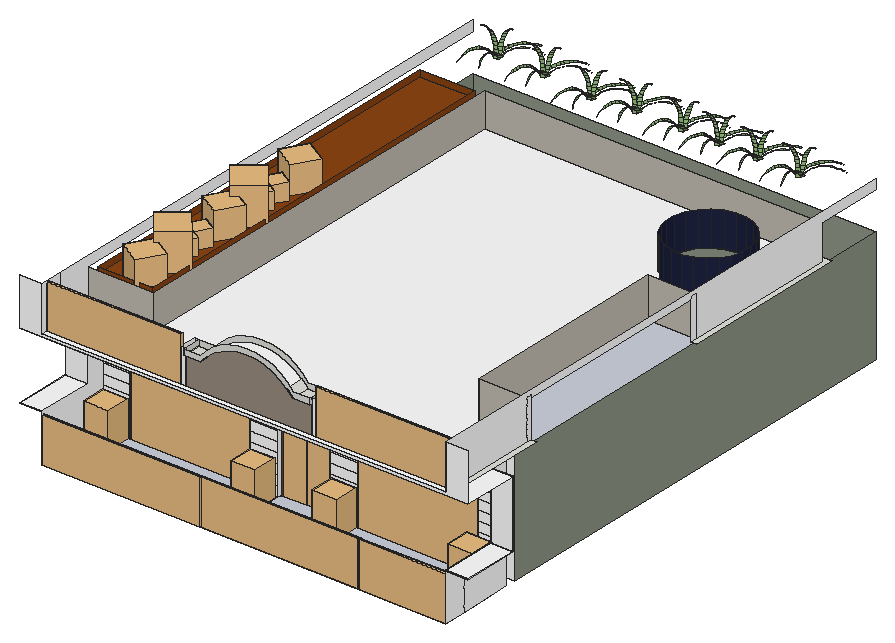
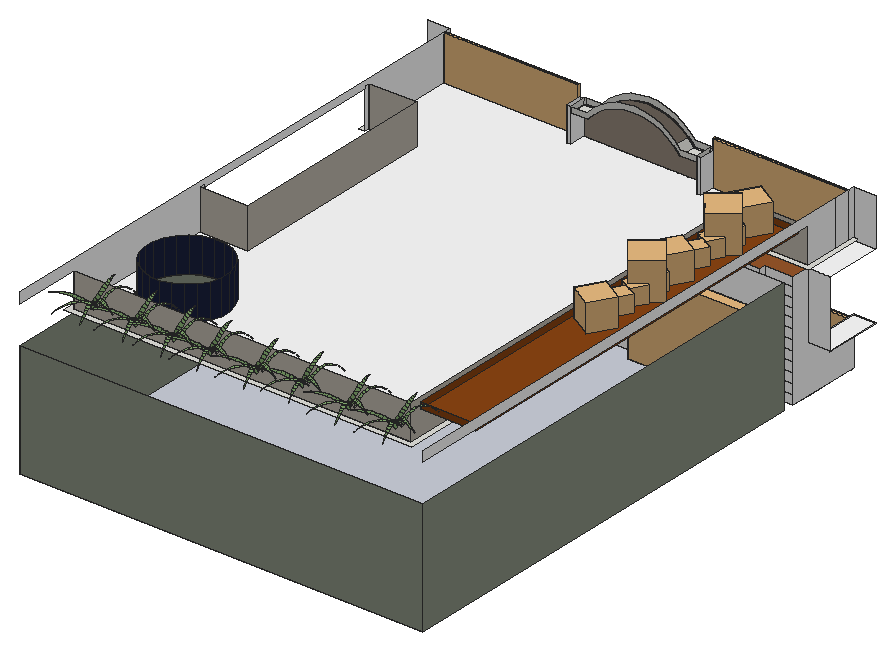
# SketchUp Ruby script. Lengths in inches.
U = 1.inch
M = Sketchup.active_model
def pt(a) = Geom::Point3d.new(a.map { |v| v * U })
def face(e, loops, mat)
  f = e.add_face(loops[0].map { |a| pt(a) })
  loops[1..].each { |l| e.add_face(l.map { |a| pt(a) }).erase! }
  f.material = f.back_material = mat if mat
  f
end
# faces: each face lists its corners as indices into pts; further lists are holes
def faces(e, pts, list, mat = nil) = list.each { |f| face(e, (f[0].is_a?(Array) ? f : [f]).map { |l| l.map { |i| pts[i] } }, mat) }
# xy, xz, yz: faces in a plane at the given z, y or x. An outline is a flat list of corners, or four numbers for a rectangle; further outlines are holes
def ring(l) = l.size == 4 ? [[l[0], l[1]], [l[2], l[1]], [l[2], l[3]], [l[0], l[3]]] : l.each_slice(2).to_a
def flat(e, list, mat, &to3) = list.each { |f| face(e, (f[0].is_a?(Array) ? f : [f]).map { |l| ring(l).map { |u, v| to3.(u, v) } }, mat) }
def xy(e, z, list, mat = nil) = flat(e, list, mat) { |x, y| [x, y, z] }
def xz(e, y, list, mat = nil) = flat(e, list, mat) { |x, z| [x, y, z] }
def yz(e, x, list, mat = nil) = flat(e, list, mat) { |y, z| [x, y, z] }
def lines(e, pts, list) = list.each { |a, b| e.add_line(pt(pts[a]), pt(pts[b])) }
# prism: a flat outline (further loops are holes) pulled along v
def prism(e, loops, v, mat = nil)
  f = face(e, loops, mat); d = Geom::Vector3d.new(v.map { |x| x * U })
  f.pushpull(f.normal.samedirection?(d) ? d.length : -d.length)
end
def box(e, o, s, mat = nil) = prism(e, [[o, [o[0] + s[0], o[1], o[2]], [o[0] + s[0], o[1] + s[1], o[2]], [o[0], o[1] + s[1], o[2]]]], [0, 0, s[2]], mat)
def at(x, y, z, deg = 0) = Geom::Transformation.translation(pt([x, y, z])) * Geom::Transformation.rotation(ORIGIN, Z_AXIS, deg.degrees)
def axes(o, x, y, z) = Geom::Transformation.new([*x, 0, *y, 0, *z, 0, *pt(o).to_a, 1])
def part(name) = M.definitions.add(name)
# library, detail: a bought-in or finely detailed component or shape, given as its bounding box
def library(name, o, s) = part(name).tap { |d| box(d.entities, o, s) }
def detail(e, o, s) = box(e.add_group.entities, o, s)
def put(e, d, t, mat = nil) = e.add_instance(d, t).tap { |i| i.material = mat if mat }
def group(e, t, mat = nil) = e.add_group.tap { |g| g.transformation = t; g.material = mat if mat }.entities
root = M.entities
M.materials.add("LAM 2").color = [91, 74, 54]
M.materials.add("LAM 2\#1").color = [121, 98, 72]
M.materials.add("W144X974F75_NILAYA EQUINOX FD25761 ROLL F75").color = [143, 150, 135]
M.materials.add("YELLOW V").color = [99, 70, 40]
M.materials.add("[0043_SaddleBrown]").color = [139, 69, 19]
M.materials.add("[0099_LightSteelBlue]").color = [176, 196, 222]
M.materials.add("[0119_RosyBrown]").color = [29, 34, 63]
M.materials.add("[Color M00]").color = [255, 255, 255]
M.materials.add("[Field Rectangle Tile]").color = [196, 189, 179]
M.materials.add("[Marble Carrara Floor Tile]").color = [204, 208, 219]
M.materials.add("[Wood Cherry Original]").color = [152, 86, 42]
M.materials.add("[Wood Floor Dark]").color = [154, 141, 128]
M.materials.add("dianella").color = [131, 171, 111]
c1 = library("Group\#437",[-4.67,-0.54,0],[25.91,25.89,38.25])
c2 = library("Group\#273",[0,-5.22,0],[72,5.22,55.56])
c3 = library("03_Wagner_Railings_Glass_Railing",[9.08,102.375,1.53],[2.51,145.5,42.05])
c4 = library("Group\#72",[0,0,0],[27.68,2.95,82.68])
c5 = part("Group\#41")
g1 = group(c5.entities,at(58.46,4.92,0,180),"YELLOW V")
xy(g1,0,[[0,0,0,4.92,1.5,4.92,1.5,3.35,1.97,3.35,1.97,0]])
xy(g1,82.2,[[1.97,0,15.59,3.35]])
xy(g1,82.68,[[1.5,3.35,15.59,4.92]])
xy(g1,84.17,[[0,0,15.59,4.92]])
xz(g1,0,[[0,0,1.97,0,1.97,82.2,15.59,82.2,15.59,84.17,0,84.17]])
xz(g1,3.35,[[1.5,0,1.5,82.68,15.59,82.68,15.59,82.2,1.97,82.2,1.97,0]])
xz(g1,4.92,[[0,0,0,84.17,1.5,82.68,1.5,0]],"LAM 2")
xz(g1,4.92,[[1.5,82.68,0,84.17,15.59,84.17,15.59,82.68]],"LAM 2\#1")
yz(g1,0,[[0,0,4.92,84.17]])
yz(g1,1.5,[[3.35,0,4.92,82.68]])
yz(g1,1.97,[[0,0,3.35,82.2]])
yz(g1,15.59,[[0,82.2,3.35,82.2,3.35,82.68,4.92,82.68,4.92,84.17,0,84.17]])
g2 = group(c5.entities,at(0.47,4.92,0),"LAM 2")
xy(g2,0,[[0,-4.92,1.5,-4.92,1.5,-3.35,1.97,-3.35,1.97,0,0,0]])
xy(g2,82.2,[[1.97,-3.35,50.39,0]])
xy(g2,82.68,[[1.5,-4.92,50.39,-3.35]])
xy(g2,84.17,[[0,-4.92,50.39,0]])
xz(g2,-4.92,[[0,0,0,84.17,1.5,82.68,1.5,0]],"LAM 2")
xz(g2,-4.92,[[1.5,82.68,0,84.17,50.39,84.17,50.39,82.68]],"LAM 2\#1")
xz(g2,-3.35,[[1.5,0,1.5,82.68,50.39,82.68,50.39,82.2,1.97,82.2,1.97,0]])
xz(g2,0,[[0,0,1.97,0,1.97,82.2,50.39,82.2,50.39,84.17,0,84.17]])
yz(g2,0,[[-4.92,0,0,84.17]])
yz(g2,1.5,[[-4.92,0,-3.35,82.68]])
yz(g2,1.97,[[-3.35,0,0,82.2]])
yz(g2,50.39,[[-3.35,82.2,-3.35,82.68,-4.92,82.68,-4.92,84.17,0,84.17,0,82.2]])
c6 = library("Group\#4",[0,0,0],[124.96,11.66,102.54])
c7 = part("Shape Bender Component\#5")
p = [[0.17,0.01,0.72],[1.09,0.03,4.5625],[1.09,3.73,4.5625],[0.17,3.75,0.72],[2.23,0.05,7.59],[2.48,0.0625,8.26],
  [2.48,3.71,8.26],[2.23,3.72,7.59],[4.33,0.14,11.74],[4.33,3.64,11.74],[6.2,0.2,14.41],[6.6,0.22,14.97],
  [6.6,3.56,14.97],[6.2,3.58,14.41],[9.26,0.35,17.88],[9.26,3.43,17.88],[12.27,0.4,20.43],[12.27,3.38,20.43],
  [15.58,0.51,22.59],[15.58,3.27,22.59],[19.13,0.73,24.3],[19.13,3.14,24.3],[22.875,1.08,25.56],[22.875,2.85,25.56],
  [26.75,1.47,26.33],[26.75,2.49,26.33],[30.68,1.86,26.6],[30.68,2.125,26.6],[33.95,1.875,26.45]]
faces(c7.entities,p,[[0,1,2,3],[1,4,5,6,7,2],[5,8,9,6],[8,10,11,12,13,9],[11,14,15,12],[14,16,17,15],[16,18,19,17],[18,20,21,19],
  [20,22,23,21],[22,24,25,23],[24,26,27,25],[28,27,26]],"dianella")
c8 = library("Group\#74",[-84.69,-90.07,-0.36],[176.51,175.13,171.4])
c9 = library("Areca palm plant",[0,0,0],[49.1,36.6,54.46])
xy(root,123,[[24,0,211.83,24],[211.83,0,267,24],[267,0,456,24]],"[Color M00]")
xy(root,123,[[24,24,211.83,60],[211.83,24,267,60],[267,24,456,60],[24,60,211.83,60,211.83,81,181.83,81,181.83,93,54,93,54,81,24,81],[211.83,60,267,93],
  [267,60,456,60,456,81,426,81,426,93,297,93,297,81,267,81],[24,93,456,576]],"[Marble Carrara Floor Tile]")
xy(root,173.5625,[[456,0,480,60]],"[Color M00]")
xy(root,174.0625,[[456,0,480,60],[456,60,480,60.3125]],"[Color M00]")
xy(root,174.75,[[0,0,24,60.9375]],"[Color M00]")
xy(root,207,[[211.83,81,267,93],[297,87.125,426,93],[54,87.375,181.83,93]],"[Color M00]")
xy(root,246.0625,[[0,0,24,60.9375],[456,0,480,60],[456,60,480,60.3125]],"[Color M00]")
xy(root,246.0625,[[24,0,24,81,54,81,54,87.375,181.83,87.375,181.83,81,297,81,297,87.125,426,87.125,426,81,456,81,456,0]],"[Wood Cherry Original]")
xy(root,249.0625,[[18,0,24,0,24,60.88,94.68,60.88,94.68,503.79,456,503.79,456,328.96,462,328.96,462,509.79,88.68,509.79,88.68,66.88,18,66.88],[456,0,462,114.58]])
xy(root,249.0625,[[24,0,456,6],[[24,6,168,6,168,24,172.5,24,172.5,6,307.5,6,307.5,24,312,24,312,6,456,6,456,108.58,405,108.58,405,334.96,456,334.96,456,503.79,94.68,503.79,94.68,60.88,24,60.88],[398.2,388.3,387.21,388.51,376.64,391.55,367.22,397.23,359.59,405.15,354.27,414.77,351.63,425.45,351.83,436.44,354.88,447.01,360.55,456.43,368.47,464.06,378.1,469.375,388.77,472.02,399.77,471.82,410.34,468.77,419.75,463.1,427.38,455.18,432.7,445.55,435.35,434.88,435.14,423.88,432.1,413.32,426.42,403.9,418.5,396.27,408.88,390.95]]],"[Color M00]")
xy(root,279.0625,[[172.5,4,190.5,6],[289.625,4,307.5,6],[172.5,6,190.5,24],[289.625,6,307.5,24]])
xy(root,279.5,[[30,66.88,88.68,497.79]],"[0043_SaddleBrown]")
xz(root,0,[[456,173.5625,480,174.0625],[0,174.0625,24,174.75],[0,246.0625,480,246.0625,480,297.0625,456,297.0625,456,249.0625,24,249.0625,24,297.0625,0,297.0625]],"[Color M00]")
xz(root,4,[[172.5,279.0625,190.5,279.0625,196.93,286.04,204.32,291.98,212.53,296.75,221.35,300.23,230.6,302.35,240.0625,303.0625,249.52,302.35,258.77,300.23,267.6,296.75,275.8,291.98,283.2,286.04,289.625,279.0625,307.5,279.0625,307.5,285.0625,289.5,285.0625,283.09,292.04,275.7,297.98,267.51,302.75,258.69,306.23,249.45,308.35,240,309.0625,230.55,308.35,221.31,306.23,212.49,302.75,204.3,297.98,196.91,292.04,190.5,285.0625,172.5,285.0625]])
xz(root,6,[[168,249.0625,172.5,285.0625],[307.5,249.0625,312,285.0625]],"[Color M00]")
xz(root,6,[[172.5,249.0625,307.5,249.0625,307.5,279.0625,289.625,279.0625,283.2,286.04,275.8,291.98,267.6,296.75,258.77,300.23,249.52,302.35,240.0625,303.0625,230.6,302.35,221.35,300.23,212.53,296.75,204.32,291.98,196.93,286.04,190.5,279.0625,172.5,279.0625]],"[Wood Floor Dark]")
xz(root,24,[[172.5,279.0625,172.5,285.0625,190.5,285.0625,196.91,292.04,204.3,297.98,212.49,302.75,221.31,306.23,230.55,308.35,240,309.0625,249.45,308.35,258.69,306.23,267.51,302.75,275.7,297.98,283.09,292.04,289.5,285.0625,307.5,285.0625,307.5,279.0625,289.625,279.0625,283.2,286.04,275.8,291.98,267.6,296.75,258.77,300.23,249.52,302.35,240.0625,303.0625,230.6,302.35,221.35,300.23,212.53,296.75,204.32,291.98,196.93,286.04,190.5,279.0625]])
xz(root,24,[[168,249.0625,172.5,285.0625],[307.5,249.0625,312,285.0625]],"[Color M00]")
xz(root,60,[[456,173.5625,480,174.0625],[456,174.0625,480,246.0625]],"[Color M00]")
xz(root,60.3125,[[456,174.0625,480,246.0625]],"[Color M00]")
xz(root,60.88,[[24,249.0625,94.68,286.25]],"[Field Rectangle Tile]")
xz(root,60.9375,[[0,174.75,24,246.0625]],"[Color M00]")
xz(root,66.88,[[30,279.5,88.68,286.25]],"[0043_SaddleBrown]")
xz(root,81,[[24,123,54,133.5],[181.83,123,211.83,133.5],[267,123,297,133.5],[426,123,456,133.5],[24,133.5,54,144],
  [181.83,133.5,211.83,144],[267,133.5,297,144],[426,133.5,456,144],[24,144,54,154.5],[181.83,144,211.83,154.5],
  [267,144,297,154.5],[426,144,456,154.5],[24,154.5,54,165],[181.83,154.5,211.83,165],[267,154.5,297,165],
  [426,154.5,456,165],[24,165,54,175.5],[181.83,165,211.83,175.5],[267,165,297,175.5],[426,165,456,175.5],
  [24,175.5,54,186],[181.83,175.5,211.83,186],[267,175.5,297,186],[426,175.5,456,186],[24,186,54,196.5],
  [181.83,186,211.83,196.5],[267,186,297,196.5],[426,186,456,196.5],[24,196.5,54,207],[181.83,196.5,211.83,207],
  [267,196.5,297,207],[426,196.5,456,207],[24,207,54,216.77],[181.83,207,211.83,216.77],[267,207,297,216.77],
  [426,207,456,216.77],[24,216.77,54,226.53],[181.83,216.77,211.83,226.53],[267,216.77,297,226.53],[426,216.77,456,226.53],
  [24,226.53,54,236.3],[181.83,226.53,211.83,236.3],[267,226.53,297,236.3],[426,226.53,456,236.3],[24,236.3,54,246.0625],
  [181.83,236.3,211.83,246.0625],[267,236.3,297,246.0625],[426,236.3,456,246.0625]],"[Color M00]")
xz(root,81,[[211.83,207,267,246.0625]],"[Wood Cherry Original]")
xz(root,87.125,[[297,207,426,246.0625]],"[Color M00]")
xz(root,87.375,[[54,207,181.83,246.0625]],"[Color M00]")
xz(root,93,[[24,123,24,246.0625,456,246.0625,456,123,426,123,426,207,297,207,297,123,267,123,267,207,211.83,207,211.83,123,181.83,123,181.83,207,54,207,54,123]],"[Color M00]")
xz(root,108.58,[[405,249.0625,456,292.1875]],"[Field Rectangle Tile]")
xz(root,334.96,[[405,249.0625,456,292.1875]],"[Field Rectangle Tile]")
xz(root,497.79,[[30,279.5,88.68,286.25]],"[0043_SaddleBrown]")
xz(root,503.79,[[94.68,249.0625,456,286.25]],"[Field Rectangle Tile]")
xz(root,576,[[24,123,456,246.0625]],"W144X974F75_NILAYA EQUINOX FD25761 ROLL F75")
yz(root,0,[[0,174.0625,60,174.75],[60,174.0625,60.9375,174.75]],"[Color M00]")
yz(root,24,[[93,123,576,246.0625]],"W144X974F75_NILAYA EQUINOX FD25761 ROLL F75")
yz(root,24,[[0,123,81,123,81,246.0625,60.9375,246.0625,60.9375,174.75,0,174.75],[0,249.0625,6,297.0625],[6,249.0625,24,297.0625],[24,249.0625,60.88,249.0625,60.88,286.25,576,286.25,576,297.0625,24,297.0625]],"[Color M00]")
yz(root,30,[[66.88,279.5,497.79,286.25]],"[0043_SaddleBrown]")
yz(root,54,[[81,123,93,123,93,207,87.375,207,87.375,246.0625,81,246.0625]],"[Color M00]")
yz(root,88.68,[[66.88,279.5,497.79,286.25]],"[0043_SaddleBrown]")
yz(root,94.68,[[60.88,249.0625,503.79,286.25]],"[Field Rectangle Tile]")
yz(root,168,[[6,249.0625,24,285.0625]],"[Color M00]")
yz(root,172.5,[[4,279.0625,6,285.0625],[6,279.0625,24,285.0625]])
yz(root,172.5,[[6,249.0625,24,279.0625]],"[Color M00]")
yz(root,181.83,[[81,123,81,246.0625,87.375,246.0625,87.375,207,93,207,93,123]],"[Color M00]")
yz(root,211.83,[[81,123,93,207]],"[Color M00]")
yz(root,267,[[81,123,93,207]],"[Color M00]")
yz(root,297,[[81,123,93,123,93,207,87.125,207,87.125,246.0625,81,246.0625]],"[Color M00]")
yz(root,307.5,[[4,279.0625,6,285.0625],[6,279.0625,24,285.0625]])
yz(root,307.5,[[6,249.0625,24,279.0625]],"[Color M00]")
yz(root,312,[[6,249.0625,24,285.0625]],"[Color M00]")
yz(root,405,[[108.58,249.0625,334.96,292.1875]],"[Field Rectangle Tile]")
yz(root,426,[[81,123,81,246.0625,87.125,246.0625,87.125,207,93,207,93,123]],"[Color M00]")
yz(root,456,[[93,123,576,246.0625]],"W144X974F75_NILAYA EQUINOX FD25761 ROLL F75")
yz(root,456,[[0,123,24,173.5625],[24,123,24,173.5625,60,173.5625,60,174.0625,60.3125,174.0625,60.3125,246.0625,81,246.0625,81,123],[0,173.5625,24,174.0625],[24,173.5625,60,174.0625],[60,174.0625,60.3125,246.0625],
  [0,249.0625,0,297.0625,576,297.0625,576,286.25,503.79,286.25,503.79,249.0625,334.96,249.0625,334.96,292.1875,328.96,292.1875,328.96,289.375,114.58,289.375,114.58,292.1875,108.58,292.1875,108.58,249.0625],[108.58,249.0625,114.58,292.1875],[328.96,249.0625,334.96,292.1875]],"[Color M00]")
yz(root,480,[[0,173.5625,60,174.0625],[60,174.0625,60.3125,246.0625]],"[Color M00]")
p = [[387.21,388.51,249.0625],[398.2,388.3,249.0625],[398.2,388.3,286.25],[387.21,388.51,286.25],[408.88,390.95,249.0625],[408.88,390.95,286.25],
  [376.64,391.55,249.0625],[376.64,391.55,286.25],[418.5,396.27,249.0625],[418.5,396.27,286.25],[367.22,397.23,249.0625],[367.22,397.23,286.25],
  [426.42,403.9,249.0625],[426.42,403.9,286.25],[359.59,405.15,249.0625],[359.59,405.15,286.25],[432.1,413.32,249.0625],[432.1,413.32,286.25],
  [354.27,414.77,249.0625],[354.27,414.77,286.25],[435.14,423.88,249.0625],[435.14,423.88,286.25],[351.63,425.45,249.0625],[351.63,425.45,286.25],
  [435.35,434.88,249.0625],[435.35,434.88,286.25],[351.83,436.44,249.0625],[351.83,436.44,286.25],[432.7,445.55,249.0625],[432.7,445.55,286.25],
  [354.88,447.01,249.0625],[354.88,447.01,286.25],[427.38,455.18,249.0625],[427.38,455.18,286.25],[360.55,456.43,249.0625],[360.55,456.43,286.25],
  [419.75,463.1,249.0625],[419.75,463.1,286.25],[368.47,464.06,249.0625],[368.47,464.06,286.25],[410.34,468.77,249.0625],[410.34,468.77,286.25],
  [378.1,469.375,249.0625],[378.1,469.375,286.25],[399.77,471.82,249.0625],[399.77,471.82,286.25],[388.77,472.02,249.0625],[388.77,472.02,286.25],
  [190.5,6,279.0625],[196.93,6,286.04],[196.93,4,286.04],[190.5,4,279.0625],[283.2,6,286.04],[289.625,6,279.0625],
  [289.625,4,279.0625],[283.2,4,286.04],[190.5,24,279.0625],[196.93,24,286.04],[283.2,24,286.04],[289.625,24,279.0625],
  [24,60,174.0625],[0,60,174.0625],[24,60.9375,174.0625],[0,60.9375,174.0625]]
faces(root,p,[[0,1,2,3],[1,4,5,2],[6,0,3,7],[4,8,9,5],[10,6,7,11],[8,12,13,9],[14,10,11,15],[12,16,17,13],
  [18,14,15,19],[16,20,21,17],[22,18,19,23],[20,24,25,21],[26,22,23,27],[24,28,29,25],[30,26,27,31],[28,32,33,29],
  [34,30,31,35],[32,36,37,33],[38,34,35,39],[36,40,41,37],[42,38,39,43],[40,44,45,41],[46,42,43,47],[44,46,47,45]],"[0119_RosyBrown]")
faces(root,p,[[48,49,50,51],[52,53,54,55],[49,48,56,57],[53,52,58,59]])
lines(root,p,[[60,61],[62,63]])
put(root,c1,at(29.86,54.9,123))
put(root,c1,at(419.64,54.27,123))
put(root,c1,at(274,55.26,123))
put(root,c1,at(189.46,52.03,123))
put(root,c2,axes([181.83,81,123],[-1.79167,0,0],[0,-1,0],[0,0,1.55963]))
put(root,c3,axes([312.41,-9.08,121.25],[0,1,0],[-1.16351,0,0],[0,0,1.14163]))
put(root,c4,axes([265.7,84.96,123],[-0.95143,0,0],[0,0.54,0],[0,0,0.99794]))
put(root,c5,axes([211.38,86.66,123],[0.95143,0,0],[0,-0.54,0],[0,0,0.99794]),"LAM 2")
put(root,c4,axes([213.0625,84.96,123],[0.95143,0,0],[0,0.54,0],[0,0,0.99794]))
put(root,c6,axes([54,93,123],[1.02301,0,0],[0,1,0],[0,0,0.86]))
put(root,c6,axes([297,93,123],[1.03237,0,0],[0,1,0],[0,0,0.86]),"[Marble Carrara Floor Tile]")
put(root,c3,axes([522.49,-9.08,121.25],[0,1,0],[-0.64948,0,0],[0,0,1.14163]),"[0099_LightSteelBlue]")
put(root,c2,axes([426,81,123],[-1.79167,0,0],[0,-0.56,0],[0,0,1.53964]))
put(root,c3,axes([481.7,-8.92,121.25],[0,1,0],[-1.16351,0,0],[0,0,1.14163]))
put(root,c3,axes([269.32,-3.08,247.33],[0,1,0],[-0.98969,0,0],[0,0,1.1323]))
put(root,c3,axes([557.15,-3.08,247.3125],[0,1,0],[-0.98899,0,0],[0,0,1.14163]))
put(root,c7,axes([122.7,545.26,291.85],[-0.344,-0.60231,-0.75479],[-0.91328,0.3827,0.2032],[-0.0732,-0.41342,1.09421]))
put(root,c7,axes([221.11,545.26,291.85],[-0.344,-0.60231,-0.75479],[-0.91328,0.3827,0.2032],[-0.0732,-0.41342,1.09421]))
put(root,c7,axes([309.58,545.26,291.85],[-0.344,-0.60231,-0.75479],[-0.91328,0.3827,0.2032],[-0.0732,-0.41342,1.09421]))
put(root,c7,axes([395.79,545.26,291.85],[-0.344,-0.60231,-0.75479],[-0.91328,0.3827,0.2032],[-0.0732,-0.41342,1.09421]))
put(root,c7,axes([177.19,539.26,291.85],[-0.344,-0.60231,-0.75479],[-0.91328,0.3827,0.2032],[-0.0732,-0.41342,1.09421]))
put(root,c7,axes([72.18,545.26,291.85],[-0.344,-0.60231,-0.75479],[-0.91328,0.3827,0.2032],[-0.0732,-0.41342,1.09421]))
put(root,c7,axes([270.67,545.26,291.85],[-0.344,-0.60231,-0.75479],[-0.91328,0.3827,0.2032],[-0.0732,-0.41342,1.09421]))
put(root,c7,axes([350.68,545.26,291.85],[-0.344,-0.60231,-0.75479],[-0.91328,0.3827,0.2032],[-0.0732,-0.41342,1.09421]))
put(root,c7,axes([121.73,546.09,291.04],[0.40267,0.75319,-0.5066],[-0.83258,0.53685,0.13638],[0.3594,0.37082,0.7344]))
put(root,c7,axes([220.14,546.09,291.04],[0.40267,0.75319,-0.5066],[-0.83258,0.53685,0.13638],[0.3594,0.37082,0.7344]))
put(root,c7,axes([308.62,546.09,291.04],[0.40267,0.75319,-0.5066],[-0.83258,0.53685,0.13638],[0.3594,0.37082,0.7344]))
put(root,c7,axes([394.82,546.09,291.04],[0.40267,0.75319,-0.5066],[-0.83258,0.53685,0.13638],[0.3594,0.37082,0.7344]))
put(root,c7,axes([176.22,540.09,291.04],[0.40267,0.75319,-0.5066],[-0.83258,0.53685,0.13638],[0.3594,0.37082,0.7344]))
put(root,c7,axes([71.21,546.09,291.04],[0.40267,0.75319,-0.5066],[-0.83258,0.53685,0.13638],[0.3594,0.37082,0.7344]))
put(root,c7,axes([269.7,546.09,291.04],[0.40267,0.75319,-0.5066],[-0.83258,0.53685,0.13638],[0.3594,0.37082,0.7344]))
put(root,c7,axes([349.71,546.09,291.04],[0.40267,0.75319,-0.5066],[-0.83258,0.53685,0.13638],[0.3594,0.37082,0.7344]))
put(root,c7,axes([124.04,546.6,292.88],[-0.25014,0.81662,-0.56232],[0.92036,0.36652,0.15138],[-0.28129,0.43308,0.81519]))
put(root,c7,axes([222.44,546.6,292.88],[-0.25014,0.81662,-0.56232],[0.92036,0.36652,0.15138],[-0.28129,0.43308,0.81519]))
put(root,c7,axes([310.92,546.6,292.88],[-0.25014,0.81662,-0.56232],[0.92036,0.36652,0.15138],[-0.28129,0.43308,0.81519]))
put(root,c7,axes([397.125,546.6,292.88],[-0.25014,0.81662,-0.56232],[0.92036,0.36652,0.15138],[-0.28129,0.43308,0.81519]))
put(root,c7,axes([178.52,540.6,292.88],[-0.25014,0.81662,-0.56232],[0.92036,0.36652,0.15138],[-0.28129,0.43308,0.81519]))
put(root,c7,axes([73.52,546.6,292.88],[-0.25014,0.81662,-0.56232],[0.92036,0.36652,0.15138],[-0.28129,0.43308,0.81519]))
put(root,c7,axes([272,546.6,292.88],[-0.25014,0.81662,-0.56232],[0.92036,0.36652,0.15138],[-0.28129,0.43308,0.81519]))
put(root,c7,axes([352.01,546.6,292.88],[-0.25014,0.81662,-0.56232],[0.92036,0.36652,0.15138],[-0.28129,0.43308,0.81519]))
put(root,c7,axes([124.82,546.71,290.01],[0.94392,0.13849,-0.29973],[-0.24231,0.89782,-0.34826],[0.18658,0.40957,0.77683]))
put(root,c7,axes([223.22,546.71,290.01],[0.94392,0.13849,-0.29973],[-0.24231,0.89782,-0.34826],[0.18658,0.40957,0.77683]))
put(root,c7,axes([311.7,546.71,290.01],[0.94392,0.13849,-0.29973],[-0.24231,0.89782,-0.34826],[0.18658,0.40957,0.77683]))
put(root,c7,axes([397.9,546.71,290.01],[0.94392,0.13849,-0.29973],[-0.24231,0.89782,-0.34826],[0.18658,0.40957,0.77683]))
put(root,c7,axes([179.3,540.71,290.01],[0.94392,0.13849,-0.29973],[-0.24231,0.89782,-0.34826],[0.18658,0.40957,0.77683]))
put(root,c7,axes([74.3,546.71,290.01],[0.94392,0.13849,-0.29973],[-0.24231,0.89782,-0.34826],[0.18658,0.40957,0.77683]))
put(root,c7,axes([272.78,546.71,290.01],[0.94392,0.13849,-0.29973],[-0.24231,0.89782,-0.34826],[0.18658,0.40957,0.77683]))
put(root,c7,axes([352.79,546.71,290.01],[0.94392,0.13849,-0.29973],[-0.24231,0.89782,-0.34826],[0.18658,0.40957,0.77683]))
put(root,c8,axes([67.42,189.53,279.53],[-0.08133,-0.14087,0],[0.14087,-0.08133,0],[0,0,0.1725]))
put(root,c8,axes([67.42,84.09,279.53],[-0.08133,-0.14087,0],[0.14087,-0.08133,0],[0,0,0.1725]))
put(root,c8,axes([67.42,291.34,279.53],[-0.08133,-0.14087,0],[0.14087,-0.08133,0],[0,0,0.1725]))
put(root,c8,axes([65.16,261.47,279.5],[-0.04961,-0.08593,0],[0.08593,-0.04961,0],[0,0,0.10522]))
put(root,c8,axes([65.16,241.41,279.5],[-0.04961,-0.08593,0],[0.08593,-0.04961,0],[0,0,0.10522]))
put(root,c8,axes([65.16,159.66,279.5],[-0.04961,-0.08593,0],[0.08593,-0.04961,0],[0,0,0.10522]))
put(root,c8,axes([65.16,214.16,279.5],[-0.04961,-0.08593,0],[0.08593,-0.04961,0],[0,0,0.10522]))
put(root,c8,axes([65.16,112.35,279.5],[-0.04961,-0.08593,0],[0.08593,-0.04961,0],[0,0,0.10522]))
put(root,c8,axes([65.16,139.6,279.5],[-0.04961,-0.08593,0],[0.08593,-0.04961,0],[0,0,0.10522]))
put(root,c9,axes([44.04,226.7,279.53],[0.45017,-0.56191,0],[0.66137,0.52986,0],[0,0,0.72]))
put(root,c9,axes([44.04,124.89,279.53],[0.45017,-0.56191,0],[0.66137,0.52986,0],[0,0,0.72]))
put(root,c7,axes([128.35,549.71,291.63],[0.41151,-0.86071,-0.31771],[-0.88035,-0.29963,-0.36915],[-0.23589,-0.3833,0.82344]))
put(root,c7,axes([226.76,549.71,291.63],[0.41151,-0.86071,-0.31771],[-0.88035,-0.29963,-0.36915],[-0.23589,-0.3833,0.82344]))
put(root,c7,axes([315.23,549.71,291.63],[0.41151,-0.86071,-0.31771],[-0.88035,-0.29963,-0.36915],[-0.23589,-0.3833,0.82344]))
put(root,c7,axes([401.4375,549.71,291.63],[0.41151,-0.86071,-0.31771],[-0.88035,-0.29963,-0.36915],[-0.23589,-0.3833,0.82344]))
put(root,c7,axes([182.84,543.71,291.63],[0.41151,-0.86071,-0.31771],[-0.88035,-0.29963,-0.36915],[-0.23589,-0.3833,0.82344]))
put(root,c7,axes([77.83,549.71,291.63],[0.41151,-0.86071,-0.31771],[-0.88035,-0.29963,-0.36915],[-0.23589,-0.3833,0.82344]))
put(root,c7,axes([276.32,549.71,291.63],[0.41151,-0.86071,-0.31771],[-0.88035,-0.29963,-0.36915],[-0.23589,-0.3833,0.82344]))
put(root,c7,axes([356.33,549.71,291.63],[0.41151,-0.86071,-0.31771],[-0.88035,-0.29963,-0.36915],[-0.23589,-0.3833,0.82344]))
put(root,c7,axes([124.22,541.82,292.45],[-0.8996,0.31763,-0.3327],[0.41063,0.83437,-0.38657],[-0.10424,0.43783,0.86228]))
put(root,c7,axes([222.62,541.82,292.45],[-0.8996,0.31763,-0.3327],[0.41063,0.83437,-0.38657],[-0.10424,0.43783,0.86228]))
put(root,c7,axes([311.1,541.82,292.45],[-0.8996,0.31763,-0.3327],[0.41063,0.83437,-0.38657],[-0.10424,0.43783,0.86228]))
put(root,c7,axes([397.3,541.82,292.45],[-0.8996,0.31763,-0.3327],[0.41063,0.83437,-0.38657],[-0.10424,0.43783,0.86228]))
put(root,c7,axes([178.7,535.82,292.45],[-0.8996,0.31763,-0.3327],[0.41063,0.83437,-0.38657],[-0.10424,0.43783,0.86228]))
put(root,c7,axes([73.7,541.82,292.45],[-0.8996,0.31763,-0.3327],[0.41063,0.83437,-0.38657],[-0.10424,0.43783,0.86228]))
put(root,c7,axes([272.18,541.82,292.45],[-0.8996,0.31763,-0.3327],[0.41063,0.83437,-0.38657],[-0.10424,0.43783,0.86228]))
put(root,c7,axes([352.19,541.82,292.45],[-0.8996,0.31763,-0.3327],[0.41063,0.83437,-0.38657],[-0.10424,0.43783,0.86228]))
